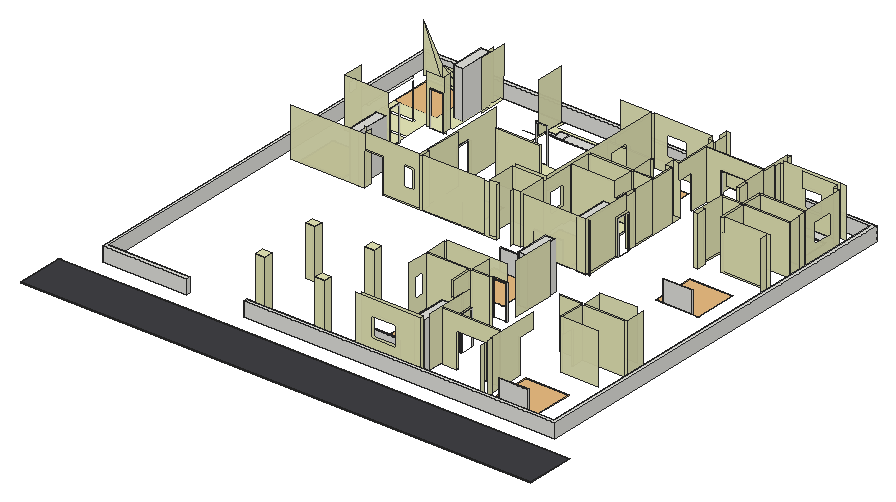
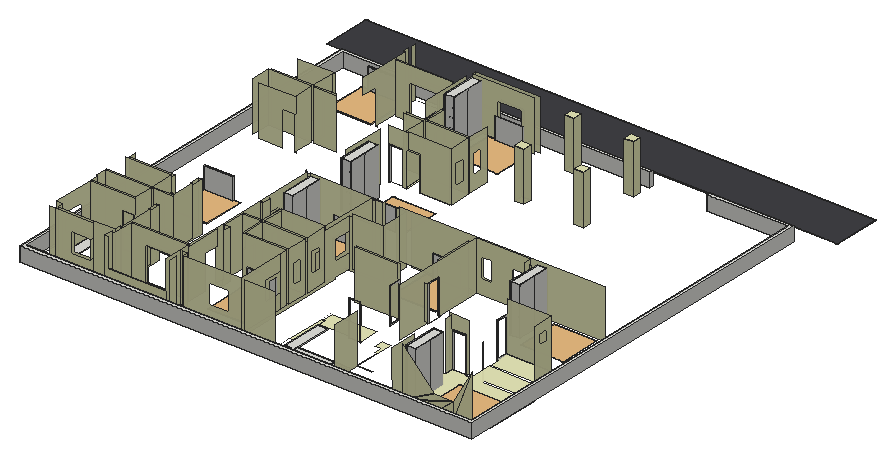
# SketchUp Ruby script. Lengths in inches.
U = 1.inch
M = Sketchup.active_model
def pt(a) = Geom::Point3d.new(a.map { |v| v * U })
def face(e, loops, mat)
  f = e.add_face(loops[0].map { |a| pt(a) })
  loops[1..].each { |l| e.add_face(l.map { |a| pt(a) }).erase! }
  f.material = f.back_material = mat if mat
  f
end
# faces: each face lists its corners as indices into pts; further lists are holes
def faces(e, pts, list, mat = nil) = list.each { |f| face(e, (f[0].is_a?(Array) ? f : [f]).map { |l| l.map { |i| pts[i] } }, mat) }
# xy, xz, yz: faces in a plane at the given z, y or x. An outline is a flat list of corners, or four numbers for a rectangle; further outlines are holes
def ring(l) = l.size == 4 ? [[l[0], l[1]], [l[2], l[1]], [l[2], l[3]], [l[0], l[3]]] : l.each_slice(2).to_a
def flat(e, list, mat, &to3) = list.each { |f| face(e, (f[0].is_a?(Array) ? f : [f]).map { |l| ring(l).map { |u, v| to3.(u, v) } }, mat) }
def xy(e, z, list, mat = nil) = flat(e, list, mat) { |x, y| [x, y, z] }
def xz(e, y, list, mat = nil) = flat(e, list, mat) { |x, z| [x, y, z] }
def yz(e, x, list, mat = nil) = flat(e, list, mat) { |y, z| [x, y, z] }
def lines(e, pts, list) = list.each { |a, b| e.add_line(pt(pts[a]), pt(pts[b])) }
# prism: a flat outline (further loops are holes) pulled along v
def prism(e, loops, v, mat = nil)
  f = face(e, loops, mat); d = Geom::Vector3d.new(v.map { |x| x * U })
  f.pushpull(f.normal.samedirection?(d) ? d.length : -d.length)
end
def box(e, o, s, mat = nil) = prism(e, [[o, [o[0] + s[0], o[1], o[2]], [o[0] + s[0], o[1] + s[1], o[2]], [o[0], o[1] + s[1], o[2]]]], [0, 0, s[2]], mat)
def at(x, y, z, deg = 0) = Geom::Transformation.translation(pt([x, y, z])) * Geom::Transformation.rotation(ORIGIN, Z_AXIS, deg.degrees)
def axes(o, x, y, z) = Geom::Transformation.new([*x, 0, *y, 0, *z, 0, *pt(o).to_a, 1])
def part(name) = M.definitions.add(name)
# library, detail: a bought-in or finely detailed component or shape, given as its bounding box
def library(name, o, s) = part(name).tap { |d| box(d.entities, o, s) }
def detail(e, o, s) = box(e.add_group.entities, o, s)
def put(e, d, t, mat = nil) = e.add_instance(d, t).tap { |i| i.material = mat if mat }
def group(e, t, mat = nil) = e.add_group.tap { |g| g.transformation = t; g.material = mat if mat }.entities
root = M.entities
M.materials.add("Asphalt Black 15-01 100cm").color = [65, 65, 69]
M.materials.add("METAL").color = [0, 0, 0]
M.materials.add("WALL PAINT").color = [233, 234, 185]
M.materials["WALL PAINT"].alpha = 0.97
c1 = library("BED",[-54,-53,-0.5],[108,106,1])
c2 = part("zw$4074")
put(c2.entities,c1,at(-177.13,-155.62,0.04,-179.97))
put(c2.entities,c1,at(-177.13,115.32,0.04,-179.97))
put(c2.entities,c1,at(145.38,-151.12,0.04,-179.97))
c3 = part("zw$FF1D")
put(c3.entities,c1,at(140.52,-153.67,0.04,-179.97))
put(c3.entities,c1,at(-181.99,-153.67,0.04,-179.97))
put(c3.entities,c1,at(-188.6,153.33,0.04,0.03))
c4 = part("zw$BB06")
put(c4.entities,c1,at(-177.75,-146.34,0.04,-179.97))
put(c4.entities,c1,at(-183.63,160.66,0.04,0.03))
put(c4.entities,c1,at(141.76,-146.34,0.04,-179.97))
c5 = part("Group\#8")
box(c5.entities,[2,0,-0.35],[20.4375,85.09,0.7])
c6 = part("Group\#9")
box(c6.entities,[-0.71,0,0],[0.71,42.55,118.58])
c7 = part("Group\#12")
box(c7.entities,[0,0,0],[72,2.96,54])
c8 = part("Group\#43")
prism(c8.entities,[[[4.5,119.95,0],[148.52,119.95,0],[148.52,105,0],[163.5,104.95,0],[163.5,0,0],[136.51,0,0],[136.51,95.02,0],[0,95.02,0],[0,104.95,0],[4.5,104.95,0]]],[0,0,1.57])
box(root,[579.88,279.9375,0.08],[24,23.99,126],"WALL PAINT")
box(root,[429.88,279.93,0.08],[24,24,126],"WALL PAINT")
box(root,[579.88,437.43,0.08],[24,24,126],"WALL PAINT")
box(root,[429.88,437.43,0.08],[24,24,126],"WALL PAINT")
xy(root,0.08,[[1202.16,1061.49,1203.13,1061.49,1203.13,1202.8,1201.95,1202.8,1201.73,1202.78,1201.52,1202.74,1201.3,1202.69,1201.1,1202.63,1200.89,1202.55,1200.69,1202.46,1200.5,1202.36,1200.14,1202.12,1199.97,1201.98,1199.81,1201.83,1199.67,1201.67,1199.53,1201.5,1199.4,1201.33,1199.18,1200.95,1199.09,1200.75,1199.02,1200.55,1198.95,1200.34,1198.87,1199.92,1198.85,1199.7,1198.84,1199.48,1198.84,1064.82,1198.85,1064.6,1198.87,1064.38,1198.95,1063.96,1199.09,1063.54,1199.18,1063.35,1199.29,1063.15,1199.4,1062.97,1199.53,1062.79,1199.67,1062.625,1199.81,1062.47,1199.97,1062.32,1200.14,1062.18,1200.32,1062.05,1200.5,1061.9375,1200.69,1061.84,1200.89,1061.75,1201.1,1061.67,1201.3,1061.61,1201.52,1061.56,1201.73,1061.52,1201.95,1061.5],[82.63,1062,87.1,1062,87.3125,1062.02,87.53,1062.06,87.74,1062.11,87.95,1062.17,88.15,1062.25,88.35,1062.34,88.54,1062.44,88.9,1062.68,89.07,1062.82,89.23,1062.97,89.375,1063.13,89.51,1063.3,89.64,1063.47,89.76,1063.66,89.86,1063.85,89.95,1064.05,90.03,1064.25,90.09,1064.46,90.14,1064.67,90.17,1064.88,90.19,1065.1,90.2,1065.32,90.2,1199.99,90.19,1200.2,90.17,1200.42,90.14,1200.63,90.09,1200.85,90.03,1201.05,89.95,1201.26,89.86,1201.45,89.76,1201.65,89.64,1201.83,89.51,1202.01,89.375,1202.18,89.23,1202.33,89.07,1202.48,88.9,1202.62,88.72,1202.75,88.54,1202.86,88.35,1202.97,87.95,1203.13,87.74,1203.19,87.53,1203.24,87.3125,1203.28,87.1,1203.3,86.88,1203.31,82.63,1203.31],[73.63,1062.54,73.63,1202.76,73.61,1202.75,73.43,1202.62,73.27,1202.48,73.11,1202.33,72.96,1202.18,72.82,1202.01,72.69,1201.83,72.58,1201.65,72.48,1201.45,72.39,1201.26,72.3125,1201.05,72.25,1200.85,72.2,1200.63,72.16,1200.42,72.14,1200.2,72.13,1199.99,72.13,1065.32,72.14,1065.1,72.16,1064.88,72.2,1064.67,72.25,1064.46,72.3125,1064.25,72.39,1064.05,72.48,1063.85,72.58,1063.66,72.69,1063.47,72.82,1063.3,72.96,1063.13,73.11,1062.97,73.27,1062.82,73.43,1062.68,73.61,1062.56]])
xy(root,0.08,[[855.11,264.93,999.11,266.93],[798.86,467.43,803.36,491.43],[798.86,495.93,798.86,555.43,810.11,555.43,810.11,550.93,803.36,550.93,803.36,495.93],[690.86,949.93,690.86,1003.93,798.86,1003.93,798.86,979.93,803.34,979.93,803.34,949.93],[118.61,949.98,118.61,1003.89,228.86,1003.89,228.86,979.89,233.34,979.89,233.34,949.98],
  [118.61,1008.39,118.61,1196.93,126.13,1196.93,126.13,1211.89,276.86,1211.89,276.86,1196.89,281.38,1196.89,281.38,1087.39,276.88,1087.39,276.88,1063.39,240.86,1063.39,240.86,1067.89,118.63,1067.89,118.63,1063.39,198.86,1063.39,198.86,1067.89,228.86,1067.89,228.86,1008.39],[690.86,1008.43,690.86,1063.43,803.34,1063.43,803.34,1033.43,798.86,1033.43,798.86,1008.43],[486.86,1038.39,486.86,1091.89,516.86,1091.89,516.86,1087.39,594.86,1087.39,594.86,1067.93,599.36,1067.93,599.36,1038.39],[603.86,1038.39,603.88,1067.93],[1056.11,1038.43,1056.11,1091.93,1086.11,1091.93,1086.11,1087.39,1167.13,1087.39,1167.13,1067.89,1171.61,1067.89,1171.61,1038.43],
  [429.86,1063.43,429.86,1168.39,393.29,1168.39,393.29,1172.89,429.86,1172.89,429.86,1242.89,285.86,1242.89,285.86,1196.89,276.86,1196.89,276.86,1211.89,149.39,1211.89,149.39,1220.89,276.86,1220.89,276.86,1244.89,438.86,1244.89,438.86,1220.93,540.86,1220.93,540.86,1211.93,453.91,1211.93,453.91,1196.93,434.36,1196.93,434.36,1106.89,438.86,1106.89,438.86,1087.43,453.91,1087.43,453.91,1063.43],[594.86,1067.93,603.88,1168.37],[603.86,1168.37,603.88,1211.89],[690.88,1211.89,721.64,1211.93]],"WALL PAINT")
xy(root,36.08,[[73.63,243.93,285.86,243.93,285.86,252.93,82.63,252.93,82.63,1247.93,1203.13,1247.93,1203.13,252.93,429.86,252.93,429.86,243.93,1212.13,243.93,1212.13,1256.93,73.63,1256.93]])
xz(root,243.93,[[73.63,0.08,285.86,36.08],[429.86,0.08,1212.13,36.08]])
xz(root,252.93,[[82.63,0.08,285.86,36.08],[429.86,0.08,1203.13,36.08]])
xz(root,279.93,[[[681.86,0.08,846.11,128.27],[722.29,38.64,782.29,86.64]]],"WALL PAINT")
xz(root,288.93,[[[690.86,0.08,846.11,128.27],[722.29,38.64,782.29,86.64]]],"WALL PAINT")
xz(root,303.93,[[1003.61,0.08,1008.11,128.27]],"WALL PAINT")
xz(root,336.93,[[855.11,0.08,891.67,0.08,891.67,86.64,962.54,86.64,962.54,0.08,999.11,0.08,999.11,128.27,855.11,128.27]],"WALL PAINT")
xz(root,341.43,[[855.11,0.08,855.11,128.27,999.11,128.27,999.11,0.08,962.54,0.08,962.54,86.64,891.67,86.64,891.67,0.08]],"WALL PAINT")
xz(root,396.93,[[999.11,0.08,1003.61,86.64]],"WALL PAINT")
xz(root,456.93,[[1057.61,0.08,1152.13,128.27]],"WALL PAINT")
xz(root,467.43,[[798.86,0.08,803.36,86.64]],"WALL PAINT")
xz(root,491.43,[[690.86,0.08,798.86,128.27],[803.36,0.08,850.63,128.27],[1057.61,0.08,1062.11,86.64]],"WALL PAINT")
xz(root,495.93,[[690.86,0.08,798.86,128.27],[803.36,0.08,855.11,128.27]],"WALL PAINT")
xz(root,521.43,[[1003.63,0.08,1057.61,128.27],[1062.11,0.08,1167.11,128.27]],"WALL PAINT")
xz(root,525.93,[[999.11,0.08,1057.61,128.27],[1062.11,0.08,1171.61,128.27]],"WALL PAINT")
xz(root,550.93,[[690.86,0.08,768.11,0.08,768.11,86.64,798.86,86.64,798.86,128.27,690.86,128.27]],"WALL PAINT")
xz(root,555.43,[[690.86,0.08,690.86,128.27,846.13,128.27,846.13,86.64,810.11,86.64,810.11,0.08,798.86,0.08,798.86,86.64,768.11,86.64,768.11,0.08]],"WALL PAINT")
xz(root,579.43,[[1057.61,0.08,1057.61,128.27,1152.11,128.27,1152.11,0.08,1092.11,0.08,1092.11,86.64,1062.11,86.64,1062.11,0.08],[1152.11,0.08,1152.13,128.27]],"WALL PAINT")
xz(root,792.43,[[[109.63,0.08,293.86,0.08,293.86,86.64,339.86,86.64,339.86,0.08,627.86,0.08,627.86,126.08,109.63,126.08],[392.97,38.64,416.97,86.64]]],"WALL PAINT")
xz(root,796.89,[[[339.86,0.08,339.86,86.64,293.86,86.64,293.86,126.08,429.86,126.08,429.86,0.08],[392.97,38.64,416.97,86.64]],[438.88,0.08,594.86,126.08]],"WALL PAINT")
xz(root,796.93,[[690.86,0.08,849.11,126.08],[855.09,0.08,861.11,126.08]],"WALL PAINT")
xz(root,801.43,[[603.86,0.08,627.86,126.08],[663.86,0.08,681.86,126.08]],"WALL PAINT")
xz(root,816.39,[[276.86,0.08,281.36,126.08]],"WALL PAINT")
xz(root,816.78,[[434.36,0.08,438.88,126.08]],"WALL PAINT")
xz(root,873.43,[[603.86,0.08,681.86,126.08]],"WALL PAINT")
xz(root,882.43,[[603.88,0.08,603.88,126.08,681.86,126.08,681.86,3.52,690.86,3.52,690.86,0.08]],"WALL PAINT")
xz(root,889.93,[[849.11,0.08,855.09,86.64]],"WALL PAINT")
xz(root,913.87,[[429.86,0.08,434.36,90.08]],"WALL PAINT")
xz(root,925.93,[[681.86,0.08,690.86,3.52]],"WALL PAINT")
xz(root,925.98,[[846.13,0.08,855.09,0.08,855.09,86.64,849.11,86.64,849.11,126.08,846.13,126.08]],"WALL PAINT")
xz(root,945.43,[[690.86,0.08,803.34,126.08]],"WALL PAINT")
xz(root,945.48,[[850.63,0.08,855.09,126.08],[855.09,0.08,855.13,122.64],[855.09,0.08,855.13,122.64]],"WALL PAINT")
xz(root,949.93,[[429.86,0.08,438.86,90.08],[690.86,0.08,690.86,126.08,798.86,126.08,798.86,86.64,803.34,86.64,803.34,0.08],[999.11,0.08,1008.11,126.08]],"WALL PAINT")
xz(root,949.98,[[118.61,0.08,118.61,126.08,228.86,126.08,228.86,90.08,233.34,90.08,233.34,0.08],[846.13,0.08,850.63,126.08]],"WALL PAINT")
xz(root,969.39,[[482.36,0.08,594.86,126.08]],"WALL PAINT")
xz(root,969.43,[[1051.625,0.08,1167.11,0.08,1167.11,126.08,1051.61,126.08,1051.61,34.64,1051.625,34.64]],"WALL PAINT")
xz(root,973.85,[[482.36,0.08,482.36,90.08,486.86,90.08,486.86,126.08,594.86,126.08,594.86,0.08]],"WALL PAINT")
xz(root,973.93,[[1003.61,0.08,1008.11,126.08]],"WALL PAINT")
xz(root,979.93,[[798.86,0.08,803.34,86.64]],"WALL PAINT")
xz(root,1003.93,[[690.86,0.08,798.86,126.08],[803.34,0.08,850.63,126.08],[1051.61,0.08,1056.11,86.64]],"WALL PAINT")
xz(root,1008.43,[[690.86,0.08,798.86,126.08],[803.34,0.08,850.63,126.08]],"WALL PAINT")
xz(root,1033.43,[[798.86,0.08,803.34,86.64]],"WALL PAINT")
xz(root,1033.93,[[1003.61,0.08,1051.61,126.08],[1056.11,0.08,1173.01,0.08,1173.02,126.08,1056.11,126.08]],"WALL PAINT")
xz(root,1038.43,[[999.11,0.08,1051.61,126.08],[1056.11,0.08,1171.61,126.08]],"WALL PAINT")
xz(root,1063.39,[[233.36,0.08,240.86,0.08,240.86,90.08,276.88,90.08,276.88,0.08,285.86,0.08,285.86,126.08,233.36,126.08],[837.16,0.08,850.63,126.08],[855.11,0.08,855.13,126.08]],"WALL PAINT")
xz(root,1063.43,[[690.86,0.08,803.34,0.08,803.34,86.64,798.86,86.64,798.86,126.08,690.86,126.08]],"WALL PAINT")
xz(root,1067.89,[[1167.13,0.08,1171.61,126.08]],"WALL PAINT")
xz(root,1067.93,[[690.86,0.08,803.34,126.08]],"WALL PAINT")
xz(root,1082.89,[[999.11,0.08,1008.13,126.08]],"WALL PAINT")
xz(root,1087.39,[[690.86,0.08,690.88,38.64],[837.16,0.08,837.16,126.08,850.61,126.08,850.61,86.64,855.11,86.64,855.11,0.08],[1086.11,0.08,1167.13,0.08,1167.13,126.08,1056.11,126.08,1056.11,86.64,1086.11,86.64]],"WALL PAINT")
xz(root,1091.93,[[1051.61,0.08,1051.61,126.08,1167.11,126.08,1167.11,0.08,1086.11,0.08,1086.11,86.64,1056.11,86.64,1056.11,0.08]],"WALL PAINT")
xz(root,1106.93,[[1003.61,0.08,1008.13,126.08]],"WALL PAINT")
xz(root,1123.43,[[850.61,0.08,855.11,86.64]],"WALL PAINT")
xz(root,1168.43,[[855.11,0.08,891.67,0.08,891.67,86.64,962.54,86.64,962.54,0.08,999.11,0.08,999.11,126.08,855.11,126.08]],"WALL PAINT")
xz(root,1172.93,[[855.13,0.08,855.13,126.08,999.11,126.08,999.11,0.08,962.54,0.08,962.54,86.64,891.67,86.64,891.67,0.08]],"WALL PAINT")
xz(root,1196.89,[[1003.61,0.08,1008.11,126.08],[1152.13,0.08,1167.11,126.08]],"WALL PAINT")
xz(root,1196.93,[[837.16,0.08,850.61,126.08]],"WALL PAINT")
xz(root,1211.89,[[1008.11,0.08,1062.11,126.08]],"WALL PAINT")
xz(root,1211.93,[[603.88,0.08,681.86,126.08],[[690.88,0.08,837.16,126.08],[721.64,38.64,769.64,86.64]],[1062.11,0.08,1152.13,0.08,1152.13,126.08,1062.11,126.08,1062.11,86.64,1110.11,86.64,1110.11,38.64,1062.11,38.64]],"WALL PAINT")
xz(root,1220.89,[[102.13,0.08,102.13,126.08,149.39,0.08],[149.39,0.08,102.13,126.08,149.39,42.08],[149.39,0.08,149.39,42.08,197.39,0.08],[197.39,0.08,149.39,42.08,276.86,0.08],[276.86,0.08,149.39,42.08,197.39,42.08],
  [276.86,0.08,197.39,42.08,276.86,126.08]],"WALL PAINT")
xz(root,1220.93,[[1152.13,0.08,1167.11,126.08]],"WALL PAINT")
xz(root,1220.98,[[[1008.11,0.08,1152.13,126.08],[1062.11,38.64,1110.11,86.64]]],"WALL PAINT")
xz(root,1242.93,[[855.13,0.08,999.11,54.08]],"WALL PAINT")
xz(root,1244.93,[[846.11,0.08,846.11,126.08,855.13,126.08,855.13,54.08,999.11,54.08,999.11,126.08,1008.11,126.08,1008.11,0.08]],"WALL PAINT")
xz(root,1247.93,[[82.63,0.08,1203.13,36.08]])
xz(root,1256.93,[[73.63,0.08,1212.13,36.08]])
yz(root,73.63,[[243.93,0.08,1256.93,36.08]])
yz(root,82.63,[[252.93,0.08,1247.93,36.08]])
yz(root,118.61,[[[949.98,0.08,1003.89,126.08],[965.03,78.08,989.03,102.08]]],"WALL PAINT")
yz(root,198.86,[[1063.39,0.08,1067.89,90.08]],"WALL PAINT")
yz(root,276.88,[[1063.39,0.08,1063.39,90.08,1067.89,90.08,1067.89,126.08,1087.39,126.08,1087.39,0.08]],"WALL PAINT")
yz(root,285.86,[[243.93,0.08,252.93,36.08]])
yz(root,285.86,[[1172.89,0.08,1242.89,0.08,1242.89,54.08,1244.89,54.08,1244.89,126.08,1172.89,126.08]],"WALL PAINT")
yz(root,293.86,[[792.43,0.08,816.39,0.08,816.39,126.08,796.89,126.08,796.89,86.64,792.43,86.64]],"WALL PAINT")
yz(root,339.86,[[792.43,0.08,796.89,86.64]],"WALL PAINT")
yz(root,429.86,[[243.93,0.08,252.93,36.08]])
yz(root,429.86,[[796.89,0.08,796.89,126.08,1038.39,126.08,1038.39,0.08,949.93,0.08,949.93,90.08,913.87,90.08,913.87,0.08],[1172.89,0.08,1172.89,126.08,1244.89,126.08,1244.89,54.08,1242.89,54.08,1242.89,0.08]],"WALL PAINT")
yz(root,434.36,[[816.78,0.08,913.87,126.08]],"WALL PAINT")
yz(root,438.88,[[796.89,0.08,816.78,126.08]],"WALL PAINT")
yz(root,603.86,[[801.43,0.08,873.43,126.08]],"WALL PAINT")
yz(root,627.86,[[792.43,0.08,801.43,126.08]],"WALL PAINT")
yz(root,663.86,[[792.25,0.08,801.43,126.08]],"WALL PAINT")
yz(root,681.86,[[801.43,0.08,873.43,126.08],[[925.93,0.08,925.93,3.52,882.43,3.52,882.43,42.08,925.93,42.08,925.93,90.08,882.43,90.08,882.43,126.08,1211.93,126.08,1211.93,0.08],[1087.39,38.64,1135.43,86.64],[1024.53,38.64,1048.53,86.64],[965.08,38.64,989.08,86.64]]],"WALL PAINT")
yz(root,690.86,[[[437.34,0.08,491.43,128.27],[456.93,38.64,480.93,86.64]],[[495.93,0.08,550.93,128.27],[512.03,38.64,536.03,86.64]],[[796.93,0.08,882.43,0.08,882.43,3.52,925.93,3.52,925.93,0.08,945.43,0.08,945.43,126.08,796.93,126.08],[882.43,42.08,925.93,90.08]],[[949.93,0.08,1003.93,126.08],[965.08,38.64,989.08,86.64]],[[1008.43,0.08,1063.43,126.08],[1024.53,38.64,1048.53,86.64]],
  [1067.93,0.08,1087.39,126.08]],"WALL PAINT")
yz(root,690.88,[[1087.39,0.08,1211.93,0.08,1211.93,126.08,1087.39,126.08,1087.39,86.64,1135.43,86.64,1135.43,38.64,1087.39,38.64]],"WALL PAINT")
yz(root,768.11,[[550.93,0.08,555.43,86.64]],"WALL PAINT")
yz(root,798.86,[[467.43,0.08,467.43,86.64,437.34,86.64,437.34,128.27,491.43,128.27,491.43,0.08],[979.93,0.08,979.93,86.64,949.93,86.64,949.93,126.08,1003.93,126.08,1003.93,0.08],[1008.43,0.08,1008.43,126.08,1063.43,126.08,1063.43,86.64,1033.43,86.64,1033.43,0.08]],"WALL PAINT")
yz(root,803.34,[[945.43,0.08,949.93,0.08,949.93,86.64,979.93,86.64,979.93,0.08,1003.93,0.08,1003.93,126.08,945.43,126.08],[1008.43,0.08,1033.43,0.08,1033.43,86.64,1063.43,86.64,1063.43,0.08,1067.93,0.08,1067.93,126.08,1008.43,126.08]],"WALL PAINT")
yz(root,803.36,[[467.43,0.08,491.43,0.08,491.43,128.27,437.34,128.27,437.34,86.64,467.43,86.64],[495.93,0.08,550.93,128.27]],"WALL PAINT")
yz(root,810.11,[[550.93,0.08,555.43,86.64]],"WALL PAINT")
yz(root,837.16,[[1063.39,0.08,1087.39,126.08],[1196.93,0.08,1211.93,126.08]],"WALL PAINT")
yz(root,846.11,[[279.93,0.08,288.93,128.27],[1220.93,0.08,1244.93,126.08]],"WALL PAINT")
yz(root,846.13,[[925.98,0.08,949.98,126.08]],"WALL PAINT")
yz(root,849.11,[[796.93,0.08,796.93,126.08,925.98,126.08,925.98,86.64,889.93,86.64,889.93,0.08]],"WALL PAINT")
yz(root,850.61,[[303.93,0.08,303.93,128.27,432.93,128.27,432.93,86.64,396.93,86.64,396.93,0.08],[574.93,0.08,684.43,128.27],[1123.43,0.08,1123.43,86.64,1087.39,86.64,1087.39,126.08,1196.93,126.08,1196.93,0.08]],"WALL PAINT")
yz(root,850.63,[[945.48,0.08,949.98,126.08],[949.98,0.08,1003.93,126.08],[1008.43,0.08,1063.39,126.08]],"WALL PAINT")
yz(root,855.09,[[796.93,0.08,889.93,0.08,889.93,86.64,925.98,86.64,925.98,0.08,945.48,0.08,945.48,126.08,796.93,126.08]],"WALL PAINT")
yz(root,855.11,[[1063.39,0.08,1087.39,0.08,1087.39,86.64,1123.43,86.64,1123.43,0.08,1168.43,0.08,1168.43,126.08,1063.39,126.08]],"WALL PAINT")
yz(root,855.13,[[945.48,0.08,1063.39,126.08],[1172.93,0.08,1196.93,126.08],[1196.93,0.08,1242.93,0.08,1242.93,54.08,1244.93,54.08,1244.93,126.08,1196.93,126.08]],"WALL PAINT")
yz(root,861.11,[[792.25,0.08,796.93,126.08]],"WALL PAINT")
yz(root,891.67,[[336.93,0.08,341.43,86.64],[1168.43,0.08,1172.93,86.64]],"WALL PAINT")
yz(root,962.54,[[336.93,0.08,341.43,86.64],[1168.43,0.08,1172.93,86.64]],"WALL PAINT")
yz(root,999.11,[[949.93,0.08,1038.43,126.08],[1082.89,0.08,1168.43,126.08],[1172.93,0.08,1242.93,126.08]],"WALL PAINT")
yz(root,1003.61,[[303.93,0.08,396.93,0.08,396.93,86.64,437.43,86.64,437.43,128.27,303.93,128.27],[973.93,0.08,1033.93,126.08],[1106.93,0.08,1196.89,126.08]],"WALL PAINT")
yz(root,1008.11,[[264.93,0.08,279.93,128.27],[288.93,0.08,303.93,128.27],[949.93,0.08,973.93,126.08],[1196.89,0.08,1211.89,126.08],[1220.98,0.08,1244.93,126.08]],"WALL PAINT")
yz(root,1008.13,[[1082.89,0.08,1106.93,126.08]],"WALL PAINT")
yz(root,1051.61,[[1003.93,0.08,1003.93,86.64,973.93,86.64,973.93,34.64,969.43,34.64,969.43,126.08,1033.93,126.08,1033.93,0.08],[1038.43,0.08,1091.93,126.08]],"WALL PAINT")
yz(root,1051.625,[[969.43,0.08,973.93,34.64]],"WALL PAINT")
yz(root,1056.11,[[1003.93,0.08,1033.93,0.08,1033.93,126.08,973.93,126.08,973.93,86.64,1003.93,86.64],[1038.43,0.08,1091.93,0.08,1091.93,86.64,1087.39,86.64,1087.39,126.08,1038.43,126.08]],"WALL PAINT")
yz(root,1057.61,[[456.93,0.08,456.93,128.27,521.43,128.27,521.43,0.08,491.43,0.08,491.43,86.64,461.43,86.64,461.43,0.08]],"WALL PAINT")
yz(root,1062.11,[[491.43,0.08,521.43,0.08,521.43,128.27,461.43,128.27,461.43,86.64,491.43,86.64],[525.93,0.08,579.43,0.08,579.43,86.64,574.93,86.64,574.93,128.27,525.93,128.27],[1211.89,0.08,1211.93,0.08,1211.93,38.64,1220.98,38.64,1220.98,86.64,1211.93,86.64,1211.93,126.08,1211.89,126.08]],"WALL PAINT")
yz(root,1086.11,[[1087.39,0.08,1091.93,86.64]],"WALL PAINT")
yz(root,1152.13,[[1196.89,0.08,1211.93,126.08],[1220.93,0.08,1220.98,126.08]],"WALL PAINT")
yz(root,1167.11,[[949.93,0.08,969.43,126.08],[[1091.93,0.08,1196.89,126.08],[1120.41,38.64,1168.41,86.64]],[1220.89,0.08,1220.93,126.08]],"WALL PAINT")
yz(root,1167.13,[[1067.89,0.08,1087.39,126.08],[1087.39,0.08,1087.43,123.39]],"WALL PAINT")
yz(root,1171.61,[[525.93,0.08,574.93,128.27],[1038.43,0.08,1067.89,126.08]],"WALL PAINT")
yz(root,1203.13,[[252.93,0.08,1247.93,36.08]])
yz(root,1212.13,[[243.93,0.08,1256.93,36.08]])
p = [[1051.625,973.93,34.64],[1051.625,973.93,86.64],[1056.11,973.93,86.64],[1056.11,973.93,126.08],[1173.01,973.94,126.08],[1173.01,973.93,0.08],
  [1051.625,973.93,0.08]]
faces(root,p,[[0,1,2,3,4,5,6]],"WALL PAINT")
put(root,c2,at(929.41,1006.55,0.54))
put(root,c3,at(362.02,1004.5625,0.54))
put(root,c4,at(930.03,489.27,0.54))
g1 = group(root,at(233.34,949.98,0.08))
prism(g1,[[[0,29.91,0],[0,29.91,90],[0,0,90],[0,0,0]],[[0,27.91,88],[0,27.91,2],[0,2,2],[0,2,88]]],[-2,0,0])
g2 = group(root,at(240.86,1063.39,0.08))
prism(g2,[[[0,0,0],[2,0,0],[2,0,88],[34.02,0,88],[34.02,0,0],[36.02,0,0],[36.02,0,90],[0,0,90]]],[0,2,0])
p = [[2,0,0],[34.02,0,0]]
lines(g2,p,[[0,1]])
g3 = group(root,at(429.86,913.87,0.08))
prism(g3,[[[0,36.0625,0],[0,34.0625,0],[0,34.0625,88],[0,2,88],[0,2,0],[0,0,0],[0,0,90],[0,36.0625,90]]],[2,0,0])
p = [[0,34.0625,0],[0,2,0]]
lines(g3,p,[[0,1]])
g4 = group(root,at(486.86,1091.89,0.08))
prism(g4,[[[30,0,0],[28,0,0],[28,0,88],[2,0,88],[2,0,0],[0,0,0],[0,0,90],[30,0,90]]],[0,-2,0])
p = [[28,0,0],[2,0,0]]
lines(g4,p,[[0,1]])
g5 = group(root,at(482.36,973.85,0.08))
prism(g5,[[[0,0,0],[0,0,90],[0,30.03,90],[0,30.03,0]],[[0,2,88],[0,2,2],[0,28.03,2],[0,28.03,88]]],[2,0,0])
g6 = group(root,at(855.09,889.93,0.08))
prism(g6,[[[0,0,0],[0,2,0],[0,2,84.5625],[0,34.05,84.5625],[0,34.05,0],[0,36.05,0],[0,36.05,86.5625],[0,0,86.5625]]],[-2,0,0])
p = [[0,2,0],[0,34.05,0]]
lines(g6,p,[[0,1]])
g7 = group(root,at(803.34,949.93,0.08))
prism(g7,[[[0,30,0],[0,30,86.5625],[0,0,86.5625],[0,0,0]],[[0,28,2],[0,2,2],[0,2,84.5625],[0,28,84.5625]]],[-2,0,0])
g8 = group(root,at(1056.11,1091.93,0.08))
prism(g8,[[[30,0,0],[28,0,0],[28,0,84.5625],[2,0,84.5625],[2,0,0],[0,0,0],[0,0,86.5625],[30,0,86.5625]]],[0,-2,0])
p = [[28,0,0],[2,0,0]]
lines(g8,p,[[0,1]])
g9 = group(root,at(1051.61,973.93,0.08))
prism(g9,[[[0,30,0],[0.02,0,0],[0.02,0,34.5625],[0.02,0,86.5625],[0,30,86.5625]],[[0,28,2],[0,28,84.5625],[0.01,2,84.5625],[0.01,2,34.5625],[0.01,2,2]]],[2,0,0])
g10 = group(root,at(891.67,1168.43,0.08))
xy(g10,0,[[0,0,70.87,2]])
xy(g10,2,[[2,0,68.87,2]])
xy(g10,84.5625,[[2,0,68.87,2]])
xy(g10,86.5625,[[0,0,70.87,2]])
xz(g10,0,[[[0,0,70.87,86.5625],[2,2,68.87,84.5625]]])
xz(g10,2,[[[0,0,70.87,86.5625],[2,2,68.87,84.5625]]],"METAL")
yz(g10,0,[[0,0,2,86.5625]])
yz(g10,2,[[0,2,2,84.5625]])
yz(g10,68.87,[[0,2,2,84.5625]])
yz(g10,70.87,[[0,0,2,86.5625]])
g11 = group(root,at(855.11,396.93,0.08))
prism(g11,[[[0,0,0],[0,2,0],[0,2,84.5625],[0,34,84.5625],[0,34,0],[0,36,0],[0,36,86.5625],[0,0,86.5625]]],[-2,0,0])
p = [[0,2,0],[0,34,0]]
lines(g11,p,[[0,1]])
g12 = group(root,at(810.11,550.93,0.08))
prism(g12,[[[0,0,0],[2,0,0],[2,0,84.5625],[34.02,0,84.5625],[34.02,0,0],[36.02,0,0],[36.02,0,86.5625],[0,0,86.5625]]],[0,2,0])
p = [[2,0,0],[34.02,0,0]]
lines(g12,p,[[0,1]])
g13 = group(root,at(252.86,796.93,0.08))
xy(g13,0,[[0,0,24,86.51]])
xy(g13,0.71,[[0,0.71,22.4375,85.8]])
xy(g13,119.29,[[0,0.71,22.4375,85.8]])
xy(g13,120,[[0,0,24,86.51]])
xz(g13,0,[[0,0,24,120]])
xz(g13,0.71,[[0,0.71,22.4375,119.29]])
xz(g13,85.8,[[0,0.71,22.4375,119.29]])
xz(g13,86.51,[[0,0,24,120]])
yz(g13,0,[[[0,0,86.51,120],[0.71,0.71,85.8,119.29]]])
yz(g13,22.4375,[[0.71,0.71,85.8,119.29]])
yz(g13,24,[[0,0,86.51,120]])
put(g13,c5,at(0,0.71,24.71))
put(g13,c5,at(0,0.71,48.62))
put(g13,c5,at(0,0.71,72.53))
put(g13,c5,at(0,0.71,96.44))
put(g13,c6,at(0,43.25,0.71))
put(g13,c6,at(0,0.71,0.71))
put(root,c7,at(466.57,797.91,0.08))
g14 = group(root,at(252.86,1124.77,0.08))
xy(g14,0,[[0,0,24,86.51]])
xy(g14,0.71,[[0,0.71,22.4375,85.8]])
xy(g14,119.29,[[0,0.71,22.4375,85.8]])
xy(g14,120,[[0,0,24,86.51]])
xz(g14,0,[[0,0,24,120]])
xz(g14,0.71,[[0,0.71,22.4375,119.29]])
xz(g14,85.8,[[0,0.71,22.4375,119.29]])
xz(g14,86.51,[[0,0,24,120]])
yz(g14,0,[[[0,0,86.51,120],[0.71,0.71,85.8,119.29]]])
yz(g14,22.4375,[[0.71,0.71,85.8,119.29]])
yz(g14,24,[[0,0,86.51,120]])
put(g14,c5,at(0,0.71,24.71))
put(g14,c5,at(0,0.71,48.62))
put(g14,c5,at(0,0.71,72.53))
put(g14,c5,at(0,0.71,96.44))
put(g14,c6,at(0,43.25,0.71))
put(g14,c6,at(0,0.71,0.71))
g15 = group(root,at(434.36,1185.06,0.08))
prism(g15,[[[0,11.875,0],[19.55,11.875,0],[19.55,26.875,0],[42,26.875,0],[42,2,0],[0,2,0]]],[0,0,1.57])
g16 = group(root,at(476.36,1184.91,0.08))
box(g16,[0,2.15,0],[93.69,24.88,1.57])
g17 = group(root,at(567.86,1091.89,0.08))
prism(g17,[[[11.99,120.05,0],[11.99,105,0],[26.99,105,0],[26.99,0,0],[2.1875,0,0],[2.1875,120.05,0]]],[0,0,1.57])
put(root,c7,at(716.3125,797.95,0.08))
put(root,c7,at(716.31,1068.89,0.08))
put(root,c7,at(1038.82,802.45,0.08))
put(root,c7,at(1035.82,289.95,0.08))
put(root,c7,at(782.375,702.92,0.08,-180))
g18 = group(root,at(825.11,796.93,0.08))
xy(g18,0,[[0,0,24,86.55]])
xy(g18,0.71,[[0,0.71,22.4375,85.85]])
xy(g18,119.29,[[0,0.71,22.4375,85.85]])
xy(g18,120,[[0,0,24,86.55]])
xz(g18,0,[[0,0,24,120]])
xz(g18,0.71,[[0,0.71,22.4375,119.29]])
xz(g18,85.85,[[0,0.71,22.4375,119.29]])
xz(g18,86.55,[[0,0,24,120]])
yz(g18,0,[[[0,0,86.55,120],[0.71,0.71,85.85,119.29]]])
yz(g18,22.4375,[[0.71,0.71,85.85,119.29]])
yz(g18,24,[[0,0,86.55,120]])
put(g18,c5,axes([0,0.71,24.71],[1,0,0],[0,1.00052,0],[0,0,1]))
put(g18,c5,axes([0,0.71,48.62],[1,0,0],[0,1.00052,0],[0,0,1]))
put(g18,c5,axes([0,0.71,72.53],[1,0,0],[0,1.00052,0],[0,0,1]))
put(g18,c5,axes([0,0.71,96.44],[1,0,0],[0,1.00052,0],[0,0,1]))
put(g18,c6,axes([0,43.28,0.71],[1,0,0],[0,1.00052,0],[0,0,1]))
put(g18,c6,axes([0,0.71,0.71],[1,0,0],[0,1.00052,0],[0,0,1]))
g19 = group(root,at(825.11,288.93,0.08))
xy(g19,0,[[0,0,24,86.55]])
xy(g19,0.71,[[0,0.71,22.4375,85.85]])
xy(g19,119.29,[[0,0.71,22.4375,85.85]])
xy(g19,120,[[0,0,24,86.55]])
xz(g19,0,[[0,0,24,120]])
xz(g19,0.71,[[0,0.71,22.4375,119.29]])
xz(g19,85.85,[[0,0.71,22.4375,119.29]])
xz(g19,86.55,[[0,0,24,120]])
yz(g19,0,[[[0,0,86.55,120],[0.71,0.71,85.85,119.29]]])
yz(g19,22.4375,[[0.71,0.71,85.85,119.29]])
yz(g19,24,[[0,0,86.55,120]])
put(g19,c5,axes([0,0.71,24.71],[1,0,0],[0,1.00052,0],[0,0,1]))
put(g19,c5,axes([0,0.71,48.62],[1,0,0],[0,1.00052,0],[0,0,1]))
put(g19,c5,axes([0,0.71,72.53],[1,0,0],[0,1.00052,0],[0,0,1]))
put(g19,c5,axes([0,0.71,96.44],[1,0,0],[0,1.00052,0],[0,0,1]))
put(g19,c6,axes([0,43.28,0.71],[1,0,0],[0,1.00052,0],[0,0,1]))
put(g19,c6,axes([0,0.71,0.71],[1,0,0],[0,1.00052,0],[0,0,1]))
put(root,c7,at(716.26,289.99,0.08))
g20 = group(root,at(822.11,617.11,0.08))
xy(g20,0,[[0,0,24,86.55]])
xy(g20,0.71,[[0,0.71,22.4375,85.85]])
xy(g20,119.29,[[0,0.71,22.4375,85.85]])
xy(g20,120,[[0,0,24,86.55]])
xz(g20,0,[[0,0,24,120]])
xz(g20,0.71,[[0,0.71,22.4375,119.29]])
xz(g20,85.85,[[0,0.71,22.4375,119.29]])
xz(g20,86.55,[[0,0,24,120]])
yz(g20,0,[[[0,0,86.55,120],[0.71,0.71,85.85,119.29]]])
yz(g20,22.4375,[[0.71,0.71,85.85,119.29]])
yz(g20,24,[[0,0,86.55,120]])
put(g20,c5,axes([0,0.71,24.71],[1,0,0],[0,1.00052,0],[0,0,1]))
put(g20,c5,axes([0,0.71,48.62],[1,0,0],[0,1.00052,0],[0,0,1]))
put(g20,c5,axes([0,0.71,72.53],[1,0,0],[0,1.00052,0],[0,0,1]))
put(g20,c5,axes([0,0.71,96.44],[1,0,0],[0,1.00052,0],[0,0,1]))
put(g20,c6,axes([0,43.28,0.71],[1,0,0],[0,1.00052,0],[0,0,1]))
put(g20,c6,axes([0,0.71,0.71],[1,0,0],[0,1.00052,0],[0,0,1]))
put(root,c8,at(1003.61,1091.93,0.08))
g21 = group(root,at(0,76.39,0.08))
prism(g21,[[[0,0,0],[0,120.84,0],[344.75,120.84,0],[1286.9,120.84,0],[1286.9,0,0]]],[0,0,1],"Asphalt Black 15-01 100cm")
